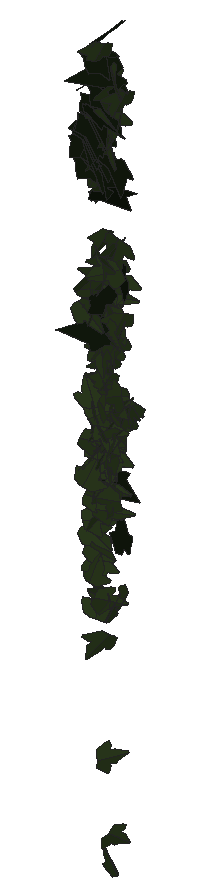
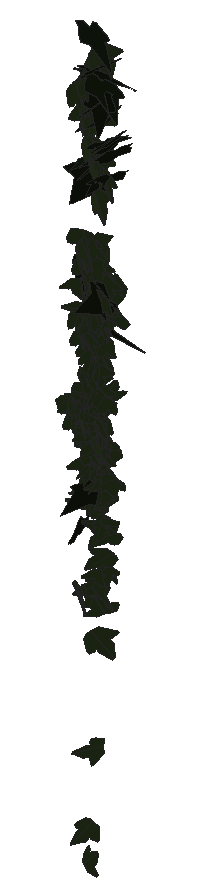
# SketchUp Ruby script. Lengths in inches.
U = 1.inch
M = Sketchup.active_model
def pt(a) = Geom::Point3d.new(a.map { |v| v * U })
def face(e, loops, mat)
  f = e.add_face(loops[0].map { |a| pt(a) })
  loops[1..].each { |l| e.add_face(l.map { |a| pt(a) }).erase! }
  f.material = f.back_material = mat if mat
  f
end
# faces: each face lists its corners as indices into pts; further lists are holes
def faces(e, pts, list, mat = nil) = list.each { |f| face(e, (f[0].is_a?(Array) ? f : [f]).map { |l| l.map { |i| pts[i] } }, mat) }
# xy, xz, yz: faces in a plane at the given z, y or x. An outline is a flat list of corners, or four numbers for a rectangle; further outlines are holes
def ring(l) = l.size == 4 ? [[l[0], l[1]], [l[2], l[1]], [l[2], l[3]], [l[0], l[3]]] : l.each_slice(2).to_a
def flat(e, list, mat, &to3) = list.each { |f| face(e, (f[0].is_a?(Array) ? f : [f]).map { |l| ring(l).map { |u, v| to3.(u, v) } }, mat) }
def xy(e, z, list, mat = nil) = flat(e, list, mat) { |x, y| [x, y, z] }
def xz(e, y, list, mat = nil) = flat(e, list, mat) { |x, z| [x, y, z] }
def yz(e, x, list, mat = nil) = flat(e, list, mat) { |y, z| [x, y, z] }
def lines(e, pts, list) = list.each { |a, b| e.add_line(pt(pts[a]), pt(pts[b])) }
# prism: a flat outline (further loops are holes) pulled along v
def prism(e, loops, v, mat = nil)
  f = face(e, loops, mat); d = Geom::Vector3d.new(v.map { |x| x * U })
  f.pushpull(f.normal.samedirection?(d) ? d.length : -d.length)
end
def box(e, o, s, mat = nil) = prism(e, [[o, [o[0] + s[0], o[1], o[2]], [o[0] + s[0], o[1] + s[1], o[2]], [o[0], o[1] + s[1], o[2]]]], [0, 0, s[2]], mat)
def at(x, y, z, deg = 0) = Geom::Transformation.translation(pt([x, y, z])) * Geom::Transformation.rotation(ORIGIN, Z_AXIS, deg.degrees)
def axes(o, x, y, z) = Geom::Transformation.new([*x, 0, *y, 0, *z, 0, *pt(o).to_a, 1])
def part(name) = M.definitions.add(name)
# library, detail: a bought-in or finely detailed component or shape, given as its bounding box
def library(name, o, s) = part(name).tap { |d| box(d.entities, o, s) }
def detail(e, o, s) = box(e.add_group.entities, o, s)
def put(e, d, t, mat = nil) = e.add_instance(d, t).tap { |i| i.material = mat if mat }
def group(e, t, mat = nil) = e.add_group.tap { |g| g.transformation = t; g.material = mat if mat }.entities
root = M.entities
M.materials.add("1026 AP 7946 SUNNY SIDE UP").color = [254, 231, 186]
M.materials.add("efeu1").color = [18, 25, 13]
M.materials.add("efeu2").color = [43, 57, 29]
c1 = part("ivyleaf_9")
p = [[1.54,2.16,1.25],[1.36,2.04,1.19],[-0.21,0.99,0.68],[-0.71,1.11,0.82],[-0.85,0.86,0.67],[-0.8,0.17,0.21],
  [-0.9,-0.01,0.1],[-0.67,-0.16,-0.02],[-0.08,-0.08,-0.05],[-0.03,-0.6,-0.4],[0.65,-0.88,-0.66],[0.83,-0.6,-0.49],
  [1.29,-0.42,-0.43],[1.8125,-0.07,-0.26],[1.21,0.44,0.15]]
faces(c1.entities,p,[[0,1,2,3,4,5,6,7,8,9,10,11,12,13,14]],"efeu1")
c2 = part("ivyleaf_10")
p = [[0,0.5,-0.03],[-0.0625,2.02,-0.43],[-0.19,2.01,-0.46],[-0.54,1.05,-0.29],[-0.52,0.625,-0.18],[-0.83,0.76,-0.28],
  [-1.16,0.64,-0.33],[-1.15,0.33,-0.24],[-0.77,-0.39,0.02],[-0.3,-0.51,0.16],[0.04,-0.48,0.23],[-0.02,2.01,-0.4375],
  [-0.06,2.01,-0.43],[0.04,-0.49,0.23],[0.67,-0.49,0.14],[1.38,0.36,-0.2],[1.375,0.51,-0.24],[0.81,0.65,-0.19],
  [0.62,0.59,-0.15],[0.6,1.09,-0.28],[0.5,1.23,-0.31]]
faces(c2.entities,p,[[0,1,2,3,4,5,6,7,8,9,10],[11,12,0,13,14,15,16,17,18,19,20]],"efeu2")
put(root,c1,axes([106.32,212.7,266.25],[-0.01839,0.24778,0.00206],[-0.05136,-0.00096,-0.25332],[-0.38621,-0.01167,0.03359]),"1026 AP 7946 SUNNY SIDE UP")
put(root,c1,axes([106.23,212.85,266.05],[0.26365,0.00517,-0.19481],[-0.29703,0.01883,-0.17189],[0.01678,0.25206,0.01832]),"1026 AP 7946 SUNNY SIDE UP")
put(root,c2,axes([106.2,213,258.72],[0.01821,-0.19998,0.03276],[0.00819,-0.03268,-0.20652],[0.31858,0.01227,0.00344]),"1026 AP 7946 SUNNY SIDE UP")
put(root,c2,axes([106.22,212.92,261.38],[-0.081,-0.21176,0.05665],[0.00013,-0.05774,-0.22443],[0.34449,-0.04977,0.0134]),"1026 AP 7946 SUNNY SIDE UP")
put(root,c2,axes([106.18,212.96,261.8],[-0.31543,0.09593,-0.04183],[0.02323,-0.06216,-0.22383],[-0.16248,-0.19512,0.04921]),"1026 AP 7946 SUNNY SIDE UP")
put(root,c1,axes([106.08,212.85,265.05],[-0.01138,-0.24732,0.02794],[-0.0061,-0.02842,-0.25504],[0.39141,-0.00763,-0.00316]),"1026 AP 7946 SUNNY SIDE UP")
put(root,c2,axes([106.23,212.89,261.43],[-0.29234,0.12636,0.02508],[-0.05554,-0.01026,-0.22982],[-0.19436,-0.18714,0.02794]),"1026 AP 7946 SUNNY SIDE UP")
put(root,c2,axes([106.09,212.57,261.75],[-0.00257,-0.14192,0.19918],[0.07029,0.19059,0.14502],[-0.37155,0.03703,0.02606]),"1026 AP 7946 SUNNY SIDE UP")
put(root,c1,axes([106.07,212.67,264.86],[0.02913,-0.22769,-0.09724],[-0.01542,0.09261,-0.23479],[0.38649,0.02085,-0.00204]),"1026 AP 7946 SUNNY SIDE UP")
put(root,c2,axes([106.21,212.71,261.31],[0.10261,-0.20388,-0.08355],[0.01101,0.08532,-0.21777],[0.34417,0.05806,0.03188]),"1026 AP 7946 SUNNY SIDE UP")
put(root,c2,axes([106.05,212.8,257.84],[-0.09375,-0.08232,-0.1819],[0.24223,0.09233,-0.09766],[0.18642,-0.16137,0.03541]),"1026 AP 7946 SUNNY SIDE UP")
put(root,c2,axes([106.24,212.96,263.92],[0.01912,-0.23668,0.00532],[-0.00531,-0.00669,-0.24416],[0.37227,0.01206,-0.00376]),"1026 AP 7946 SUNNY SIDE UP")
put(root,c2,axes([106.25,212.83,258.75],[0.02016,-0.20097,-0.0812],[-0.00075,0.07779,-0.20696],[0.33879,0.01213,0.00438]),"1026 AP 7946 SUNNY SIDE UP")
put(root,c1,axes([106.07,212.81,264.4],[0.05023,-0.20973,-0.13151],[0.01175,0.12831,-0.21652],[0.38491,0.02345,0.02377]),"1026 AP 7946 SUNNY SIDE UP")
put(root,c2,axes([106.05,212.92,261.16],[0.17272,-0.14029,-0.14093],[0.16027,-0.09197,0.182],[-0.26212,-0.14868,0.01842]),"1026 AP 7946 SUNNY SIDE UP")
put(root,c1,axes([106.09,212.84,265.14],[0.02059,-0.24901,0.02047],[-0.00015,-0.02132,-0.257],[0.39296,0.01304,-0.00117]),"1026 AP 7946 SUNNY SIDE UP")
put(root,c1,axes([106.18,212.85,265.1],[-0.13953,-0.23116,0.02196],[-0.00233,-0.02366,-0.25511],[0.3652,-0.08847,0.00676]),"1026 AP 7946 SUNNY SIDE UP")
put(root,c1,axes([106.125,212.79,261.72],[0.12039,0.12852,0.19875],[0.1977,0.14676,-0.15184],[-0.30509,0.14582,-0.01996]),"1026 AP 7946 SUNNY SIDE UP")
put(root,c1,axes([106.53,212.58,260.96],[-0.3061,0.09886,0.12154],[-0.18133,0.03095,-0.22363],[-0.15928,-0.22522,0.02102]),"1026 AP 7946 SUNNY SIDE UP")
put(root,c2,axes([106.34,212.76,262.04],[-0.33487,-0.03644,0.06432],[-0.08581,-0.04729,-0.21976],[0.07497,-0.21689,0.03575]),"1026 AP 7946 SUNNY SIDE UP")
put(root,c2,axes([106.22,212.97,259.08],[0.22596,-0.14784,-0.03854],[0.01064,0.05643,-0.20729],[0.23923,0.13713,0.04562]),"1026 AP 7946 SUNNY SIDE UP")
put(root,c2,axes([106.25,212.87,261.62],[-0.32979,0.09005,-0.01027],[0.00097,-0.02499,-0.23413],[-0.14255,-0.20851,0.02216]),"1026 AP 7946 SUNNY SIDE UP")
put(root,c2,axes([106.15,212.57,257.67],[0.33216,-0.04008,-0.03313],[0.05865,0.02738,0.21896],[-0.05526,-0.21188,0.03326]),"1026 AP 7946 SUNNY SIDE UP")
put(root,c2,axes([106.09,212.9375,259.66],[0.29918,-0.03708,0.09506],[0.15194,0.02005,-0.19641],[0.03821,0.2106,0.03671]),"1026 AP 7946 SUNNY SIDE UP")
put(root,c2,axes([106.21,212.94,257.88],[0.00264,0.1817,-0.09323],[-0.0062,-0.09149,-0.1877],[-0.31984,0.00327,0.00287]),"1026 AP 7946 SUNNY SIDE UP")
put(root,c2,axes([106.3,212.6875,264.3125],[0.26759,-0.15401,-0.08722],[-0.06264,0.07975,-0.2339],[0.26847,0.17211,0.03236]),"1026 AP 7946 SUNNY SIDE UP")
put(root,c2,axes([106.22,212.96,258.93],[0.20713,-0.15533,0.0477],[0.05221,-0.0337,-0.20998],[0.24986,0.1358,0.00433]),"1026 AP 7946 SUNNY SIDE UP")
put(root,c2,axes([106.23,212.82,260.82],[-0.3174,0.06472,-0.05778],[0.07333,-0.03849,-0.21746],[-0.11339,-0.20604,0.02111]),"1026 AP 7946 SUNNY SIDE UP")
put(root,c2,axes([106.4,212.82,259.74],[-0.31163,-0.0069,0.08813],[-0.13057,-0.03933,-0.2016],[0.03432,-0.21226,0.03321]),"1026 AP 7946 SUNNY SIDE UP")
put(root,c2,axes([106.23,212.82,255.84],[0.22273,0.15781,-0.03689],[-0.02402,-0.03553,-0.2183],[-0.25363,0.14195,-0.01172]),"1026 AP 7946 SUNNY SIDE UP")
put(root,c2,axes([106.27,212.76,256.89],[-0.05267,-0.17332,-0.13649],[0.05384,0.1272,-0.18094],[0.33783,-0.04729,0.00756]),"1026 AP 7946 SUNNY SIDE UP")
put(root,c2,axes([106.27,212.77,257.66],[0.06342,-0.16669,-0.15104],[0.04597,0.15078,-0.16852],[0.34503,0.01055,0.05022]),"1026 AP 7946 SUNNY SIDE UP")
put(root,c2,axes([106.29,212.75,261.93],[-0.16233,-0.19496,-0.04127],[0.05738,0.02457,-0.22614],[0.3073,-0.10757,0.02043]),"1026 AP 7946 SUNNY SIDE UP")
put(root,c2,axes([106.3125,212.54,259.45],[0.15549,0.19802,-0.00344],[-0.02233,0.01206,0.22733],[0.31064,-0.09825,0.01806]),"1026 AP 7946 SUNNY SIDE UP")
put(root,c2,axes([106.35,212.74,266.91],[-0.12049,-0.23479,0.0792],[-0.01337,-0.07933,-0.25438],[0.3889,-0.07547,0.01579]),"1026 AP 7946 SUNNY SIDE UP")
put(root,c2,axes([106.04,212.6,261.32],[0.21063,0.01261,0.19391],[0.29648,-0.00513,-0.13797],[-0.00492,0.23091,-0.0123]),"1026 AP 7946 SUNNY SIDE UP")
put(root,c2,axes([106.17,212.75,256.17],[0.12324,0.09874,0.1658],[0.1012,0.14921,-0.12617],[-0.27832,0.09798,0.02754]),"1026 AP 7946 SUNNY SIDE UP")
put(root,c2,axes([106.34,213,258.58],[-0.16015,-0.16447,0.0649],[-0.00204,-0.07312,-0.19633],[0.27745,-0.09547,0.03602]),"1026 AP 7946 SUNNY SIDE UP")
put(root,c2,axes([106.22,212.79,258.26],[-0.04427,-0.1565,-0.13083],[0.06631,-0.12911,0.1546],[-0.309,-0.00528,0.05192]),"1026 AP 7946 SUNNY SIDE UP")
put(root,c2,axes([106.2,212.95,261.44],[-0.18556,-0.12864,-0.14665],[0.18665,0.08127,-0.17747],[0.23594,-0.16547,0.02506]),"1026 AP 7946 SUNNY SIDE UP")
put(root,c2,axes([106.35,212.97,258.27],[0.12266,0.18492,0.04157],[-0.03071,-0.03441,0.2065],[0.29567,-0.08029,0.0042]),"1026 AP 7946 SUNNY SIDE UP")
put(root,c1,axes([106.17,212.8125,265.6],[0.05145,-0.24931,0.03048],[0.00125,-0.03116,-0.25921],[0.39504,0.03257,-0.00315]),"1026 AP 7946 SUNNY SIDE UP")
put(root,c2,axes([106.37,212.58,258.89],[-0.25849,0.11668,0.04577],[-0.06913,0.01348,-0.20709],[-0.18334,-0.16958,0.01355]),"1026 AP 7946 SUNNY SIDE UP")
put(root,c2,axes([106.36,212.85,262.87],[-0.03975,-0.20402,0.11292],[0.00996,-0.11199,-0.21166],[0.3649,-0.01917,0.01808]),"1026 AP 7946 SUNNY SIDE UP")
put(root,c2,axes([106.36,212.7,264.625],[-0.01905,-0.2338,-0.07434],[0.02206,0.07013,-0.24056],[0.3835,-0.01565,0.01014]),"1026 AP 7946 SUNNY SIDE UP")
put(root,c2,axes([106.3,212.96,260.29],[-0.21649,0.15042,-0.07681],[0.03225,-0.08171,-0.20696],[-0.26261,-0.13404,0.0379]),"1026 AP 7946 SUNNY SIDE UP")
put(root,c2,axes([106.09,212.72,258.47],[-0.06093,-0.03355,-0.22653],[0.34463,0.03118,-0.04455],[0.0579,-0.2209,0.02677]),"1026 AP 7946 SUNNY SIDE UP")
put(root,c2,axes([106.53,212.62,255.28],[0.07017,-0.06804,-0.2195],[-0.23042,0.15473,-0.08177],[0.26494,0.15259,-0.01298]),"1026 AP 7946 SUNNY SIDE UP")
put(root,c2,axes([106.45,212.74,254.34],[-0.14064,-0.18428,0.13186],[-0.07367,-0.12057,-0.21153],[0.34599,-0.10058,0.00856]),"1026 AP 7946 SUNNY SIDE UP")
put(root,c2,axes([106.31,212.65,259.3125],[-0.06157,0.21789,-0.01032],[-0.00495,-0.01199,-0.22807],[-0.34303,-0.03893,0.00514]),"1026 AP 7946 SUNNY SIDE UP")
put(root,c2,axes([106.18,212.65,256.59],[0.17026,0.12173,0.14491],[0.15153,0.10157,-0.16721],[-0.24924,0.14491,-0.00267]),"1026 AP 7946 SUNNY SIDE UP")
put(root,c2,axes([106.4,212.89,260.15],[-0.17,-0.18752,0.01875],[-0.00505,-0.02038,-0.22298],[0.29636,-0.10791,0.00696]),"1026 AP 7946 SUNNY SIDE UP")
put(root,c2,axes([106.36,213.02,258.8125],[0.25048,0.10642,-0.07427],[-0.07523,-0.05849,-0.19656],[-0.18818,0.16505,-0.02028]),"1026 AP 7946 SUNNY SIDE UP")
put(root,c2,axes([106.29,212.58,255.67],[0.31762,-0.08303,0.00112],[0.01564,0.02827,0.22303],[-0.12964,-0.20001,0.02967]),"1026 AP 7946 SUNNY SIDE UP")
put(root,c2,axes([106.32,212.85,258.24],[0.28656,0.08818,-0.01775],[-0.01255,-0.02405,-0.20787],[-0.14087,0.18152,-0.01758]),"1026 AP 7946 SUNNY SIDE UP")
put(root,c2,axes([106.33,212.91,259.73],[-0.09122,0.20807,-0.01467],[0.00535,-0.01506,-0.22261],[-0.32802,-0.05811,0.00045]),"1026 AP 7946 SUNNY SIDE UP")
put(root,c2,axes([106.15,212.6875,256.79],[0.09231,-0.03208,-0.21462],[0.29314,0.10845,0.03758],[0.15407,-0.18712,0.05708]),"1026 AP 7946 SUNNY SIDE UP")
put(root,c2,axes([106.5,212.81,257.5],[-0.23599,-0.0888,0.10644],[-0.11743,-0.07583,-0.17847],[0.17989,-0.166,0.02313]),"1026 AP 7946 SUNNY SIDE UP")
put(root,c2,axes([106.4,212.98,258.95],[0.30431,-0.04796,-0.04734],[-0.06807,0.0152,-0.20527],[0.07883,0.19827,0.00551]),"1026 AP 7946 SUNNY SIDE UP")
put(root,c1,axes([106.21,212.59,265.65],[0.30851,-0.12108,-0.08618],[-0.0568,0.09441,-0.2294],[0.2237,0.19096,0.0606]),"1026 AP 7946 SUNNY SIDE UP")
put(root,c2,axes([106.41,212.85,261.9],[0.04257,-0.22015,0.05431],[0.00945,-0.05364,-0.22882],[0.35629,0.02773,-0.00042]),"1026 AP 7946 SUNNY SIDE UP")
put(root,c2,axes([106.46,212.83,259.88],[-0.13427,-0.16998,0.09861],[-0.03415,-0.0966,-0.19529],[0.30558,-0.08548,0.0215]),"1026 AP 7946 SUNNY SIDE UP")
put(root,c2,axes([106.33,212.65,254.9],[0.21061,0.14516,-0.11361],[0.08246,0.10143,0.20225],[0.27535,-0.14141,0.02633]),"1026 AP 7946 SUNNY SIDE UP")
put(root,c1,axes([106.65,212.78,266.45],[-0.36266,0.01449,0.09808],[-0.15105,-0.04901,-0.23254],[0.00878,-0.24463,0.05091]),"1026 AP 7946 SUNNY SIDE UP")
put(root,c2,axes([106.4375,212.71,261.91],[-0.30656,-0.1097,0.00505],[0.0092,-0.0216,-0.22951],[0.17247,-0.19384,0.02121]),"1026 AP 7946 SUNNY SIDE UP")
put(root,c2,axes([106.4,212.85,260.27],[-0.09681,0.20433,0.06515],[-0.04943,0.05524,-0.21908],[-0.33213,-0.06778,0.01361]),"1026 AP 7946 SUNNY SIDE UP")
put(root,c2,axes([106.375,212.93,261.37],[-0.01087,-0.12451,-0.22558],[0.07853,0.2133,-0.12574],[0.38722,-0.04675,0.01917]),"1026 AP 7946 SUNNY SIDE UP")
put(root,c2,axes([106.42,212.88,261.25],[-0.2658,-0.14934,0.02148],[0.04173,-0.06149,-0.22338],[0.23359,-0.15895,0.06434]),"1026 AP 7946 SUNNY SIDE UP")
put(root,c1,axes([106.22,212.81,266.71],[0.12857,-0.21343,-0.11332],[0.02418,0.11939,-0.2287],[0.37591,0.06532,0.05347]),"1026 AP 7946 SUNNY SIDE UP")
put(root,c1,axes([106.58,212.73,267.34],[-0.12083,0.24311,-0.02063],[-0.00082,-0.02261,-0.26269],[-0.38374,-0.0765,0.00706]),"1026 AP 7946 SUNNY SIDE UP")
put(root,c1,axes([106.66,212.47,261.7],[-0.09934,0.16212,0.19504],[-0.13534,0.16809,-0.17776],[-0.36664,-0.10598,0.01278]),"1026 AP 7946 SUNNY SIDE UP")
put(root,c2,axes([106.48,212.78,260.53],[-0.30684,-0.08555,0.03285],[-0.01627,-0.05514,-0.21469],[0.1429,-0.18997,0.04609]),"1026 AP 7946 SUNNY SIDE UP")
put(root,c2,axes([106.44,212.72,258.27],[-0.01303,-0.13793,-0.15543],[0.02435,0.14936,-0.14141],[0.3196,-0.01701,0.00444]),"1026 AP 7946 SUNNY SIDE UP")
put(root,c2,axes([106.4,212.95,258.04],[-0.05828,0.19958,0.02634],[-0.00544,0.02421,-0.20898],[-0.31611,-0.03721,-0.00126]),"1026 AP 7946 SUNNY SIDE UP")
put(root,c2,axes([106.42,212.89,260.44],[-0.13264,-0.19086,-0.06429],[0.07681,0.04495,-0.21311],[0.30572,-0.0941,0.02565]),"1026 AP 7946 SUNNY SIDE UP")
put(root,c2,axes([106.28,212.58,257.375],[0.07914,0.06652,0.20777],[0.14041,0.18099,-0.08356],[-0.30235,0.10147,0.01558]),"1026 AP 7946 SUNNY SIDE UP")
put(root,c2,axes([106.42,212.85,264.58],[0.07311,-0.21437,0.12265],[0.05681,-0.11512,-0.22643],[0.3823,0.0581,0.01019]),"1026 AP 7946 SUNNY SIDE UP")
put(root,c2,axes([106.48,212.9375,264.98],[0.01863,-0.24263,0.02261],[0,-0.02335,-0.25039],[0.38327,0.01179,-0.0011]),"1026 AP 7946 SUNNY SIDE UP")
put(root,c2,axes([106.53,212.84,262.36],[-0.29131,-0.14047,0.03672],[-0.03322,-0.03236,-0.23934],[0.22575,-0.18602,0.01217]),"1026 AP 7946 SUNNY SIDE UP")
put(root,c1,axes([106.32,212.88,265.87],[0.07915,-0.2444,-0.03215],[-0.00167,0.03022,-0.25683],[0.38714,0.0501,0.00546]),"1026 AP 7946 SUNNY SIDE UP")
put(root,c2,axes([106.51,212.92,258.48],[-0.09939,0.08964,0.18317],[0.01459,-0.18451,0.09844],[0.31204,0.03718,0.05374]),"1026 AP 7946 SUNNY SIDE UP")
put(root,c2,axes([106.34,212.72,260.44],[0.27466,-0.07255,0.11719],[0.15998,-0.0524,-0.19498],[0.14016,0.20198,-0.00708]),"1026 AP 7946 SUNNY SIDE UP")
put(root,c2,axes([106.48,212.77,257.47],[-0.10097,-0.191,-0.0834],[0.06507,0.0701,-0.20654],[0.31896,-0.07476,0.01573]),"1026 AP 7946 SUNNY SIDE UP")
put(root,c2,axes([106.64,212.62,257.33],[0.05603,-0.02143,-0.23177],[-0.17403,0.19678,-0.03624],[0.3096,0.11449,0.02157]),"1026 AP 7946 SUNNY SIDE UP")
put(root,c1,axes([106.4,212.75,264.65],[-0.05672,-0.23862,0.0287],[-0.00113,-0.02943,-0.24877],[0.37801,-0.0359,0.00356]),"1026 AP 7946 SUNNY SIDE UP")
put(root,c2,axes([106.27,212.82,257.55],[-0.08111,-0.06249,-0.20661],[0.30846,0.05853,-0.07056],[0.11662,-0.19828,0.04292]),"1026 AP 7946 SUNNY SIDE UP")
put(root,c2,axes([106.49,212.9375,259.08],[-0.32695,-0.0002,-0.02178],[0.03315,-0.01825,-0.21349],[-0.00259,-0.2082,0.01751]),"1026 AP 7946 SUNNY SIDE UP")
put(root,c2,axes([106.625,212.77,249.46],[-0.19198,0.11281,-0.1288],[-0.12332,0.09945,0.17105],[0.23516,0.14425,-0.01544]),"1026 AP 7946 SUNNY SIDE UP")
put(root,c1,axes([106.39,212.91,257.61],[0.01582,-0.06347,-0.2442],[-0.04792,0.23472,-0.06481],[0.38232,0.03205,0.00198]),"1026 AP 7946 SUNNY SIDE UP")
put(root,c2,axes([106.28,212.95,261.51],[-0.00599,0.01021,0.2319],[0.2401,0.1656,-0.00411],[-0.26044,0.15244,-0.00912]),"1026 AP 7946 SUNNY SIDE UP")
put(root,c2,axes([106.73,212.65,262.31],[-0.21566,0.0419,0.18109],[-0.26796,-0.10265,-0.11253],[0.09342,-0.19771,0.09528]),"1026 AP 7946 SUNNY SIDE UP")
put(root,c2,axes([106.46,212.94,258.08],[0.03935,0.18875,-0.07653],[-0.0113,-0.07506,-0.19657],[-0.31937,0.02591,-0.00248]),"1026 AP 7946 SUNNY SIDE UP")
put(root,c2,axes([106.52,212.85,261.77],[-0.01189,-0.21529,-0.06974],[0.03367,0.06553,-0.22074],[0.35269,-0.01351,0.01873]),"1026 AP 7946 SUNNY SIDE UP")
put(root,c2,axes([106.51,212.6,259.41],[-0.05022,0.18751,0.1105],[-0.04923,0.10218,-0.19497],[-0.33525,-0.04309,0.01208]),"1026 AP 7946 SUNNY SIDE UP")
put(root,c2,axes([106.5,212.96,258.14],[0.23563,0.13196,-0.04194],[-0.05803,-0.02077,-0.20563],[-0.20961,0.15409,0.00978]),"1026 AP 7946 SUNNY SIDE UP")
put(root,c2,axes([106.74,212.86,259.56],[0.04739,0.00245,-0.21974],[-0.31187,-0.07902,-0.03026],[-0.12354,0.20042,-0.00789]),"1026 AP 7946 SUNNY SIDE UP")
put(root,c2,axes([106.4,212.84,258.55],[0.29665,0.02771,0.07375],[0.11511,-0.00921,-0.19557],[-0.03553,0.20152,-0.01787]),"1026 AP 7946 SUNNY SIDE UP")
put(root,c2,axes([106.79,212.58,257.48],[-0.09006,0.03373,0.21368],[-0.32774,-0.03492,-0.0537],[0.03963,-0.21214,0.04151]),"1026 AP 7946 SUNNY SIDE UP")
put(root,c2,axes([106.5,212.73,258.57],[0.31368,-0.05128,0.00866],[0.00539,-0.02142,-0.21133],[0.08161,0.19853,-0.01931]),"1026 AP 7946 SUNNY SIDE UP")
put(root,c2,axes([106.5625,212.95,260.91],[0.29882,-0.11066,-0.02666],[-0.04263,0.00356,-0.22627],[0.17331,0.19168,-0.0097]),"1026 AP 7946 SUNNY SIDE UP")
put(root,c2,axes([106.58,212.74,265.54],[-0.33996,-0.11968,-0.01141],[0.03031,-0.01343,-0.25373],[0.18644,-0.21604,0.02044]),"1026 AP 7946 SUNNY SIDE UP")
put(root,c2,axes([106.38,212.53,259.18],[0.12984,0.04007,-0.20813],[0.23959,0.13493,0.09242],[0.21843,-0.17182,0.02235]),"1026 AP 7946 SUNNY SIDE UP")
put(root,c2,axes([106.66,212.8,258.76],[-0.15919,-0.13334,0.14075],[-0.07046,-0.13459,-0.16937],[0.29267,-0.10493,0.03578]),"1026 AP 7946 SUNNY SIDE UP")
put(root,c2,axes([106.58,212.93,258.97],[0.07292,-0.20313,0.03094],[0.00608,-0.0311,-0.2148],[0.32309,0.04643,-0.00294]),"1026 AP 7946 SUNNY SIDE UP")
put(root,c2,axes([106.35,212.68,262.375],[-0.10253,0.02117,0.23805],[0.33418,-0.09058,0.06984],[0.14598,0.22223,0.00731]),"1026 AP 7946 SUNNY SIDE UP")
put(root,c2,axes([106.625,212.85,262.72],[-0.0113,-0.2351,0.02565],[0.00131,-0.02627,-0.24246],[0.37197,-0.00705,0.00163]),"1026 AP 7946 SUNNY SIDE UP")
put(root,c2,axes([106.56,212.87,259.3],[0.32457,-0.0412,-0.00216],[-0.00893,-0.019,-0.216],[0.06423,0.20555,-0.01914]),"1026 AP 7946 SUNNY SIDE UP")
put(root,c2,axes([106.41,212.98,258.73],[0.25223,0.03127,0.12973],[0.19733,0.01236,-0.16801],[-0.05076,0.20345,-0.00851]),"1026 AP 7946 SUNNY SIDE UP")
put(root,c2,axes([106.65,212.78,259.28],[-0.05205,0.10049,0.2165],[-0.11891,0.19553,-0.10774],[-0.34559,-0.08241,0.00446]),"1026 AP 7946 SUNNY SIDE UP")
put(root,c2,axes([106.71,212.67,258.35],[0.17692,-0.11958,-0.14169],[-0.12403,0.11289,-0.16775],[0.25746,0.13655,0.01656]),"1026 AP 7946 SUNNY SIDE UP")
put(root,c2,axes([106.64,212.95,262.7],[0.04597,-0.22771,0.00379],[0.00211,-0.00485,-0.23654],[0.35813,0.02926,0.00091]),"1026 AP 7946 SUNNY SIDE UP")
put(root,c2,axes([106.68,212.75,260.75],[-0.23989,-0.16145,0.0306],[-0.01451,-0.0333,-0.22843],[0.25798,-0.152,0.01561]),"1026 AP 7946 SUNNY SIDE UP")
put(root,c2,axes([106.51,212.6,251.875],[0.01839,-0.01165,-0.24591],[0.19026,0.20631,-0.00306],[0.32394,-0.12051,0.01576]),"1026 AP 7946 SUNNY SIDE UP")
put(root,c2,axes([106.56,212.65,258.9],[0.17577,0.19344,0.00439],[0.01738,-0.00274,-0.2299],[-0.30371,0.1118,-0.01062]),"1026 AP 7946 SUNNY SIDE UP")
put(root,c2,axes([106.73,212.78,262.86],[-0.3552,0.03427,0.06029],[-0.09913,-0.0329,-0.23181],[-0.03858,-0.23097,0.04056]),"1026 AP 7946 SUNNY SIDE UP")
put(root,c2,axes([106.7,212.77,258.78],[-0.07273,-0.16629,0.11459],[-0.03517,-0.11013,-0.17832],[0.31344,-0.05094,0.00658]),"1026 AP 7946 SUNNY SIDE UP")
put(root,c1,axes([106.55,212.8,264.36],[-0.02871,-0.19806,0.14338],[-0.01196,-0.14016,-0.20568],[0.38146,-0.0193,0.00435]),"1026 AP 7946 SUNNY SIDE UP")
put(root,c2,axes([106.55,212.81,260.52],[-0.08526,0.02711,-0.21332],[0.0944,-0.20304,-0.04474],[-0.31477,-0.06824,0.04436]),"1026 AP 7946 SUNNY SIDE UP")
put(root,c2,axes([106.7,212.6875,266.17],[-0.06801,-0.25572,0.0116],[-0.00036,-0.01286,-0.26725],[0.40259,-0.04321,0.00172]),"1026 AP 7946 SUNNY SIDE UP")
put(root,c2,axes([106.61,212.75,250.22],[-0.10647,-0.12907,-0.17733],[0.13063,0.14994,-0.14925],[0.31105,-0.10715,0.00198]),"1026 AP 7946 SUNNY SIDE UP")
put(root,c2,axes([106.73,212.94,258.99],[-0.23056,-0.14055,0.03001],[-0.01739,-0.03159,-0.20886],[0.22528,-0.14628,0.01459]),"1026 AP 7946 SUNNY SIDE UP")
put(root,c2,axes([106.54,212.51,255.34],[-0.08014,-0.07532,-0.21085],[0.22123,0.14867,-0.09178],[0.26119,-0.14903,0.01305]),"1026 AP 7946 SUNNY SIDE UP")
put(root,c2,axes([106.48,212.78,264.93],[0.13516,-0.10368,0.21056],[0.27373,-0.11338,-0.13495],[0.23565,0.19118,0.03599]),"1026 AP 7946 SUNNY SIDE UP")
put(root,c2,axes([106.5,212.7,261.03],[-0.12323,0.0495,-0.21842],[0.21715,-0.16329,-0.0927],[-0.26522,-0.15669,0.02559]),"1026 AP 7946 SUNNY SIDE UP")
put(root,c2,axes([106.45,212.65,257.14],[-0.00558,-0.02449,-0.22156],[0.32422,0.06461,-0.01072],[0.10285,-0.20502,0.02175]),"1026 AP 7946 SUNNY SIDE UP")
put(root,c2,axes([106.66,212.93,261.98],[0.21573,0.17567,-0.03928],[-0.04604,-0.02676,-0.22969],[-0.27923,0.14013,0.00752]),"1026 AP 7946 SUNNY SIDE UP")
put(root,c2,axes([106.9,212.58,259.73],[-0.12694,0.11236,0.17697],[-0.28944,0.0407,-0.11673],[-0.14091,-0.1848,0.08036]),"1026 AP 7946 SUNNY SIDE UP")
put(root,c2,axes([106.74,212.875,261.22],[-0.14854,-0.19752,0.06049],[0.00441,-0.06704,-0.22377],[0.32449,-0.08951,0.03074]),"1026 AP 7946 SUNNY SIDE UP")
put(root,c2,axes([106.72,212.9,261.04],[0.14244,-0.20174,-0.04242],[0.00111,0.04405,-0.22678],[0.3234,0.0887,0.01946]),"1026 AP 7946 SUNNY SIDE UP")
put(root,c2,axes([106.74,212.96,259.3],[0.23729,0.13633,-0.0541],[-0.10387,-0.00487,-0.20558],[-0.20538,0.15997,0.04147]),"1026 AP 7946 SUNNY SIDE UP")
put(root,c2,axes([106.78,212.89,255.32],[0.13174,-0.19017,-0.06918],[-0.05859,0.05568,-0.21345],[0.31109,0.09102,-0.0109]),"1026 AP 7946 SUNNY SIDE UP")
put(root,c2,axes([106.6875,212.88,258.6],[0.04809,-0.08116,0.19692],[0.07794,-0.18525,-0.09007],[0.31778,0.05772,-0.00771]),"1026 AP 7946 SUNNY SIDE UP")
put(root,c2,axes([106.7,212.71,266.5],[-0.11241,0.24323,0.00403],[-0.01325,0.00016,-0.26104],[-0.38224,-0.07153,0.00787]),"1026 AP 7946 SUNNY SIDE UP")
put(root,c1,axes([106.91,212.76,262.2],[0.03959,-0.02729,-0.2537],[-0.37128,0.07185,-0.03268],[0.11725,0.23673,-0.0178]),"1026 AP 7946 SUNNY SIDE UP")
put(root,c2,axes([106.9,212.97,259.36],[-0.23342,-0.07626,0.1332],[-0.16507,-0.07807,-0.1715],[0.16952,-0.18103,0.01641]),"1026 AP 7946 SUNNY SIDE UP")
put(root,c2,axes([106.73,212.53,255],[0.10066,-0.16992,0.12504],[-0.05873,0.11662,0.18767],[-0.32396,-0.07394,0.00483]),"1026 AP 7946 SUNNY SIDE UP")
put(root,c2,axes([106.79,212.9,259.25],[-0.10435,-0.19427,0.02551],[-0.00622,-0.02598,-0.21159],[0.3081,-0.06632,0.00437]),"1026 AP 7946 SUNNY SIDE UP")
put(root,c2,axes([106.81,212.83,266],[-0.10778,-0.23403,0.06478],[-0.01346,-0.06435,-0.25141],[0.38135,-0.06841,0.00943]),"1026 AP 7946 SUNNY SIDE UP")
put(root,c2,axes([106.77,212.78,265.65],[0.1605,-0.21148,-0.10259],[-0.00723,0.10554,-0.23802],[0.36668,0.09465,0.04021]),"1026 AP 7946 SUNNY SIDE UP")
put(root,c2,axes([106.79,212.97,259.37],[-0.00686,-0.21,0.02036],[-0.00044,-0.02095,-0.21651],[0.33185,-0.00437,0.00013]),"1026 AP 7946 SUNNY SIDE UP")
put(root,c2,axes([106.77,212.99,259.3],[-0.28416,0.10113,-0.00518],[-0.00381,-0.01576,-0.21288],[-0.15921,-0.18011,0.01432]),"1026 AP 7946 SUNNY SIDE UP")
put(root,c1,axes([106.63,212.85,264.55],[0.00753,-0.22841,0.08582],[0.02145,-0.08424,-0.23558],[0.38241,0.00922,0.01152]),"1026 AP 7946 SUNNY SIDE UP")
put(root,c1,axes([106.85,212.79,256.4375],[-0.10044,-0.12775,0.20624],[0.11694,0.18692,0.14788],[-0.35565,0.09754,-0.00962]),"1026 AP 7946 SUNNY SIDE UP")
put(root,c1,axes([106.68,212.45,264.07],[0.28296,0.1591,0.0272],[0.05102,0.00166,-0.24657],[-0.24817,0.18174,-0.01968]),"1026 AP 7946 SUNNY SIDE UP")
